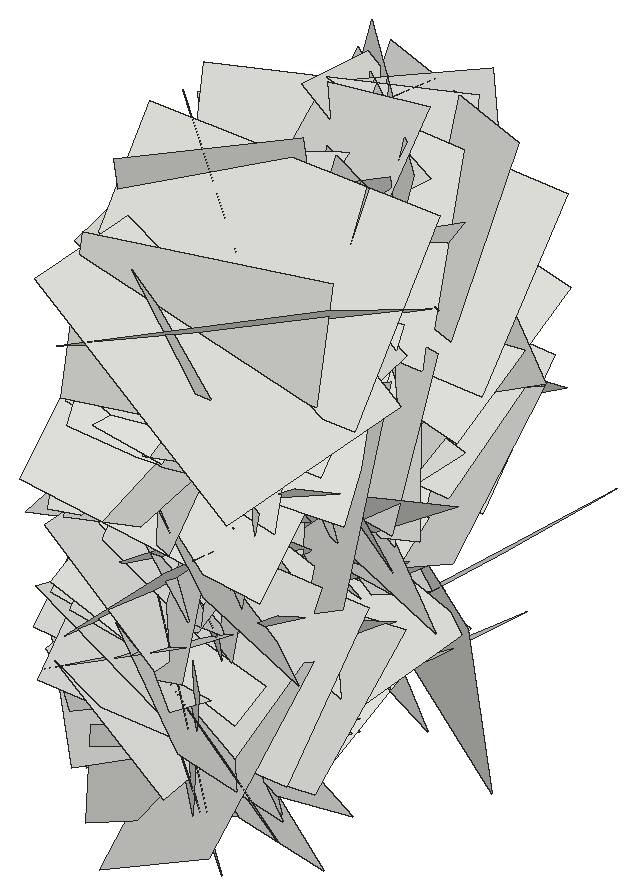
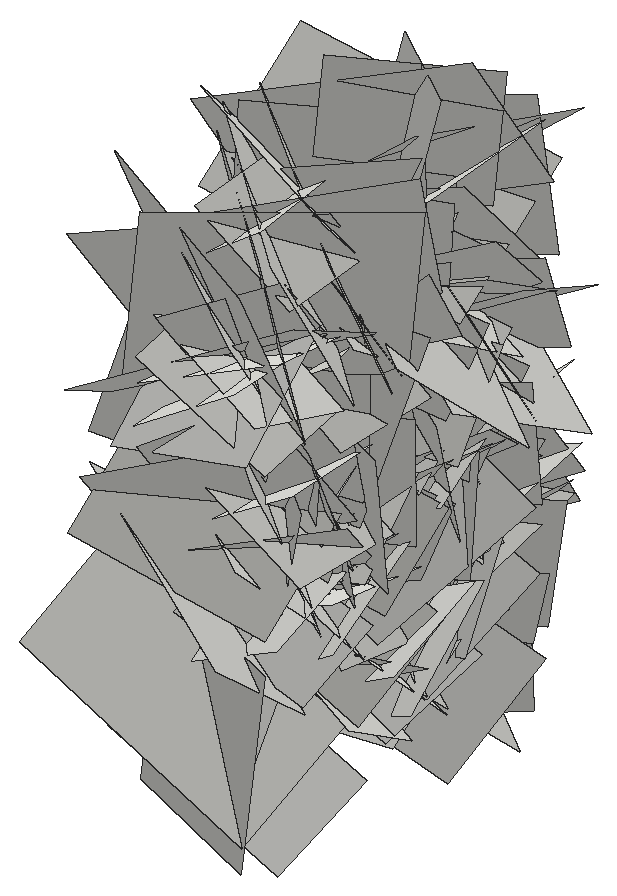
# SketchUp Ruby script. Lengths in inches.
U = 1.inch
M = Sketchup.active_model
def pt(a) = Geom::Point3d.new(a.map { |v| v * U })
def face(e, loops, mat)
  f = e.add_face(loops[0].map { |a| pt(a) })
  loops[1..].each { |l| e.add_face(l.map { |a| pt(a) }).erase! }
  f.material = f.back_material = mat if mat
  f
end
# faces: each face lists its corners as indices into pts; further lists are holes
def faces(e, pts, list, mat = nil) = list.each { |f| face(e, (f[0].is_a?(Array) ? f : [f]).map { |l| l.map { |i| pts[i] } }, mat) }
# xy, xz, yz: faces in a plane at the given z, y or x. An outline is a flat list of corners, or four numbers for a rectangle; further outlines are holes
def ring(l) = l.size == 4 ? [[l[0], l[1]], [l[2], l[1]], [l[2], l[3]], [l[0], l[3]]] : l.each_slice(2).to_a
def flat(e, list, mat, &to3) = list.each { |f| face(e, (f[0].is_a?(Array) ? f : [f]).map { |l| ring(l).map { |u, v| to3.(u, v) } }, mat) }
def xy(e, z, list, mat = nil) = flat(e, list, mat) { |x, y| [x, y, z] }
def xz(e, y, list, mat = nil) = flat(e, list, mat) { |x, z| [x, y, z] }
def yz(e, x, list, mat = nil) = flat(e, list, mat) { |y, z| [x, y, z] }
def lines(e, pts, list) = list.each { |a, b| e.add_line(pt(pts[a]), pt(pts[b])) }
# prism: a flat outline (further loops are holes) pulled along v
def prism(e, loops, v, mat = nil)
  f = face(e, loops, mat); d = Geom::Vector3d.new(v.map { |x| x * U })
  f.pushpull(f.normal.samedirection?(d) ? d.length : -d.length)
end
def box(e, o, s, mat = nil) = prism(e, [[o, [o[0] + s[0], o[1], o[2]], [o[0] + s[0], o[1] + s[1], o[2]], [o[0], o[1] + s[1], o[2]]]], [0, 0, s[2]], mat)
def at(x, y, z, deg = 0) = Geom::Transformation.translation(pt([x, y, z])) * Geom::Transformation.rotation(ORIGIN, Z_AXIS, deg.degrees)
def axes(o, x, y, z) = Geom::Transformation.new([*x, 0, *y, 0, *z, 0, *pt(o).to_a, 1])
def part(name) = M.definitions.add(name)
# library, detail: a bought-in or finely detailed component or shape, given as its bounding box
def library(name, o, s) = part(name).tap { |d| box(d.entities, o, s) }
def detail(e, o, s) = box(e.add_group.entities, o, s)
def put(e, d, t, mat = nil) = e.add_instance(d, t).tap { |i| i.material = mat if mat }
def group(e, t, mat = nil) = e.add_group.tap { |g| g.transformation = t; g.material = mat if mat }.entities
root = M.entities
c1 = part("Component\#6")
p = [[0.01,0,0],[0,3.24,4.54],[4.32,3.24,4.54],[4.33,0,0]]
faces(c1.entities,p,[[0,1,2,3]])
put(root,c1,axes([34.14,168.24,29.62],[-0.00844,-0.1319,-0.59476],[-0.00779,-0.59475,0.132],[0.64572,-0.0089,-0.00618]))
put(root,c1,axes([34.14,163.79,31.02],[-0.0186,-0.39942,0.51021],[-0.04828,0.50989,0.39761],[0.68514,0.02509,0.04187]))
put(root,c1,axes([34.14,167.3,30.05],[-0.09755,-0.36279,0.79394],[-0.2327,0.7823,0.33203],[0.89554,0.16375,0.17276]))
put(root,c1,axes([34.14,166.74,28.03],[-0.20581,0.5378,0.53941],[0.0447,0.5634,-0.54654],[0.80617,0.10606,0.16802]))
put(root,c1,axes([34.14,165.16,26.22],[0.00662,-0.41647,0.48084],[-0.04981,0.47925,0.41571],[0.67246,0.0396,0.02606]))
put(root,c1,axes([38.11,162.15,25.43],[0.09766,0.84172,-0.54191],[-0.18116,-0.52299,-0.84139],[-1.04557,0.16923,0.09516]))
put(root,c1,axes([34.14,170.38,37.22],[-0.01844,-0.65259,0.06973],[-0.0154,0.07012,0.65262],[0.69551,-0.01575,0.0163]))
put(root,c1,axes([38.11,159.15,32.85],[0.28722,0.93511,0.86971],[0.00467,0.88838,-0.95656],[-1.35365,0.20148,0.18123]))
put(root,c1,axes([34.14,158.35,30.49],[-0.08461,0.81055,-0.03501],[-0.12527,-0.04642,-0.80528],[0.85081,0.07377,-0.12204]))
put(root,c1,axes([34.14,168.23,31.98],[-0.11552,-0.73847,0.10601],[0.00435,0.10653,0.74638],[0.79079,-0.10846,0.01138]))
put(root,c1,axes([34.14,162.33,29.83],[-0.22776,0.38392,-0.75072],[0.01782,-0.77261,-0.39993],[0.89361,0.11326,-0.18337]))
put(root,c1,axes([38.11,165.04,27.71],[0.04822,0.07219,0.94774],[-0.14201,0.93984,-0.06516],[-0.99746,-0.13032,0.05509]))
put(root,c1,axes([34.14,171.91,32.4],[0.07209,-0.36069,-0.54144],[-0.07785,-0.54516,0.35394],[0.6852,-0.024,0.09718]))
put(root,c1,axes([38.11,167.29,35.58],[-0.17595,-0.29467,-0.74084],[-0.05215,-0.7515,0.30993],[-0.84352,0.10793,0.13537]))
put(root,c1,axes([38.11,157.3125,32.29],[0.25179,1.05256,0.51222],[-0.06429,0.53303,-1.06718],[-1.23914,0.18623,0.15945]))
put(root,c1,axes([34.14,168.82,35.84],[0.04533,0.37689,0.51175],[-0.01637,0.51337,-0.3768],[0.67349,-0.01289,-0.04361]))
put(root,c1,axes([34.14,159.46,22.85],[-0.09982,-0.0635,0.89488],[-0.1784,0.88507,0.04509],[0.93408,0.16225,0.10424]))
put(root,c1,axes([34.14,160.06,22.6],[-0.02839,-0.24478,0.77995],[-0.15528,0.76918,0.23637],[0.85248,0.13195,0.06903]))
put(root,c1,axes([34.14,159.67,28.14],[-0.12868,0.67272,0.52517],[-0.08613,0.51893,-0.68352],[0.90053,0.14576,0.00967]))
put(root,c1,axes([34.14,158.39,26.84],[-0.02686,0.84806,0.10272],[-0.17857,0.09579,-0.83237],[0.88773,0.04493,-0.16432]))
put(root,c1,axes([34.14,169.17,27.35],[0.00515,-0.4485,-0.48712],[0.04455,-0.48594,0.44784],[0.70046,0.0342,-0.02491]))
put(root,c1,axes([38.11,161.79,25.53],[-0.01152,-0.82607,0.19056],[-0.15176,0.18963,0.81386],[-0.88572,-0.02175,-0.14193]))
put(root,c1,axes([38.11,164.2,31.01],[0.06613,-0.18181,-0.96198],[-0.02897,-0.96387,0.1804],[-1.03734,0.01533,-0.06637]))
put(root,c1,axes([34.14,169.92,30.86],[0.08798,0.07784,-0.70174],[-0.08853,-0.70052,-0.08758],[0.74315,-0.09267,0.07264]))
put(root,c1,axes([38.11,162.32,28.44],[-0.12821,-0.42216,-0.69512],[0.01339,-0.70366,0.42514],[-0.86197,0.05186,0.11]))
put(root,c1,axes([38.11,166.33,22.3],[0.05809,-0.87115,0.26873],[-0.09257,0.26296,0.87026],[-0.96191,-0.07791,-0.06752]))
put(root,c1,axes([38.11,171.77,39.47],[0.25632,-0.1505,-1.28885],[0.2021,-1.29268,0.18672],[-1.36053,-0.22038,-0.21508]))
put(root,c1,axes([34.14,167.69,34.89],[0.01272,-0.59445,-0.3878],[0.01652,-0.38754,0.59453],[0.75216,0.01856,-0.0065]))
put(root,c1,axes([34.14,168.18,25.35],[0.0356,-0.79141,-0.13903],[-0.13499,-0.14264,0.78117],[0.84098,0.01061,0.13127]))
put(root,c1,axes([38.11,163.85,33.45],[0.03445,-0.73428,-0.4148],[-0.17499,-0.41262,0.71747],[-0.87664,0.05351,-0.15952]))
put(root,c1,axes([38.11,158.45,30.92],[0.16236,0.46297,0.88251],[-0.09478,0.89566,-0.45434],[-1.05211,-0.00924,0.17712]))
put(root,c1,axes([38.11,166.53,31.68],[0.02185,0.89564,-0.0065],[-0.05171,-0.00537,-0.89456],[-0.948,0.02094,0.04865]))
put(root,c1,axes([38.11,171.21,38.93],[0.24063,-0.51313,-1.11059],[0.16085,-1.10901,0.54342],[-1.28679,-0.23458,-0.13976]))
put(root,c1,axes([34.14,171.89,34.33],[-0.10287,-0.74562,-0.1631],[0.15609,-0.17961,0.73351],[0.79385,-0.06131,-0.16536]))
put(root,c1,axes([38.11,162.43,26.35],[-0.02315,-0.70596,0.51236],[0.01203,0.51225,0.70629],[-0.92456,0.02434,-0.00364]))
put(root,c1,axes([38.11,162.61,28.57],[0.04222,-0.49534,0.62953],[-0.20196,0.60636,0.48917],[-0.82474,-0.17384,-0.08755]))
put(root,c1,axes([38.11,162.92,24.26],[-0.16568,0.16434,-0.80239],[0.1251,-0.80382,-0.18763],[-0.85913,-0.14874,0.12742]))
put(root,c1,axes([38.11,164.5,23.79],[-0.04443,0.667,0.37408],[-0.11412,0.36576,-0.66423],[-0.80255,-0.08894,0.07374]))
put(root,c1,axes([38.11,168.875,35.8],[-0.07444,0.7996,-0.0855],[-0.00091,-0.0859,-0.80263],[-0.85241,-0.06974,0.00832]))
put(root,c1,axes([34.14,164.96,33.58],[0.03363,-0.67551,-0.53197],[-0.14584,-0.52946,0.66412],[0.89967,-0.06058,0.12754]))
put(root,c1,axes([34.14,169.82,24.93],[0.00586,-0.68753,0.27068],[0.05817,0.27032,0.6855],[0.78107,-0.01497,-0.05308]))
put(root,c1,axes([38.11,164.8,26.41],[-0.06555,-0.88967,-0.10275],[0.1194,-0.1099,0.88381],[-0.94178,0.04799,0.1192]))
put(root,c1,axes([38.11,163.99,40.83],[-0.08038,0.23372,-0.81219],[0.10222,-0.80774,-0.24144],[-0.89001,-0.11388,0.04562]))
put(root,c1,axes([38.11,167.51,23.32],[0.04127,-0.8056,0.43064],[0.05085,0.43224,0.80425],[-0.96695,-0.01165,0.06068]))
put(root,c1,axes([38.11,164.95,29.96],[0.04265,0.57286,-0.52342],[-0.15347,-0.50938,-0.56862],[-0.80809,0.12697,0.08036]))
put(root,c1,axes([34.14,164.95,29.96],[-0.04265,0.57286,-0.52342],[0.15347,-0.50938,-0.56862],[0.80809,0.12697,0.08036]))
put(root,c1,axes([34.14,167.51,23.32],[-0.04127,-0.8056,0.43064],[-0.05085,0.43224,0.80425],[0.96695,-0.01165,0.06068]))
put(root,c1,axes([34.14,163.99,40.83],[0.08038,0.23372,-0.81219],[-0.10222,-0.80774,-0.24144],[0.89001,-0.11388,0.04562]))
put(root,c1,axes([34.14,164.8,26.41],[0.06555,-0.88967,-0.10275],[-0.1194,-0.1099,0.88381],[0.94178,0.04799,0.1192]))
put(root,c1,axes([38.11,169.82,24.93],[-0.00586,-0.68753,0.27068],[-0.05817,0.27032,0.6855],[-0.78107,-0.01497,-0.05308]))
put(root,c1,axes([38.11,164.96,33.58],[-0.03363,-0.67551,-0.53197],[0.14584,-0.52946,0.66412],[-0.89967,-0.06058,0.12754]))
put(root,c1,axes([34.14,168.875,35.8],[0.07444,0.7996,-0.0855],[0.00091,-0.0859,-0.80263],[0.85241,-0.06974,0.00832]))
put(root,c1,axes([34.14,164.5,23.79],[0.04443,0.667,0.37408],[0.11412,0.36576,-0.66423],[0.80255,-0.08894,0.07374]))
put(root,c1,axes([34.14,162.92,24.26],[0.16568,0.16434,-0.80239],[-0.1251,-0.80382,-0.18763],[0.85913,-0.14874,0.12742]))
put(root,c1,axes([34.14,162.61,28.57],[-0.04222,-0.49534,0.62953],[0.20196,0.60636,0.48917],[0.82474,-0.17384,-0.08755]))
put(root,c1,axes([34.14,162.43,26.35],[0.02315,-0.70596,0.51236],[-0.01203,0.51225,0.70629],[0.92456,0.02434,-0.00364]))
put(root,c1,axes([38.11,171.89,34.33],[0.10287,-0.74562,-0.1631],[-0.15609,-0.17961,0.73351],[-0.79385,-0.06131,-0.16536]))
put(root,c1,axes([34.14,171.21,38.93],[-0.24063,-0.51313,-1.11059],[-0.16085,-1.10901,0.54342],[1.28679,-0.23458,-0.13976]))
put(root,c1,axes([34.14,166.53,31.68],[-0.02185,0.89564,-0.0065],[0.05171,-0.00537,-0.89456],[0.948,0.02094,0.04865]))
put(root,c1,axes([34.14,158.45,30.92],[-0.16236,0.46297,0.88251],[0.09478,0.89566,-0.45434],[1.05211,-0.00924,0.17712]))
put(root,c1,axes([34.14,163.85,33.45],[-0.03445,-0.73428,-0.4148],[0.17499,-0.41262,0.71747],[0.87664,0.05351,-0.15952]))
put(root,c1,axes([38.11,168.18,25.35],[-0.0356,-0.79141,-0.13903],[0.13499,-0.14264,0.78117],[-0.84098,0.01061,0.13127]))
put(root,c1,axes([38.11,167.69,34.89],[-0.01272,-0.59445,-0.3878],[-0.01652,-0.38754,0.59453],[-0.75216,0.01856,-0.0065]))
put(root,c1,axes([34.14,171.77,39.47],[-0.25632,-0.1505,-1.28885],[-0.2021,-1.29268,0.18672],[1.36053,-0.22038,-0.21508]))
put(root,c1,axes([34.14,166.33,22.3],[-0.05809,-0.87115,0.26873],[0.09257,0.26296,0.87026],[0.96191,-0.07791,-0.06752]))
put(root,c1,axes([34.14,162.32,28.44],[0.12821,-0.42216,-0.69512],[-0.01339,-0.70366,0.42514],[0.86197,0.05186,0.11]))
put(root,c1,axes([38.11,169.92,30.86],[-0.08798,0.07784,-0.70174],[0.08853,-0.70052,-0.08758],[-0.74315,-0.09267,0.07264]))
put(root,c1,axes([34.14,164.2,31.01],[-0.06613,-0.18181,-0.96198],[0.02897,-0.96387,0.1804],[1.03734,0.01533,-0.06637]))
put(root,c1,axes([34.14,161.79,25.53],[0.01152,-0.82607,0.19056],[0.15176,0.18963,0.81386],[0.88572,-0.02175,-0.14193]))
put(root,c1,axes([38.11,169.17,27.35],[-0.00515,-0.4485,-0.48712],[-0.04455,-0.48594,0.44784],[-0.70046,0.0342,-0.02491]))
put(root,c1,axes([38.11,158.39,26.84],[0.02686,0.84806,0.10272],[0.17857,0.09579,-0.83237],[-0.88773,0.04493,-0.16432]))
put(root,c1,axes([38.11,159.67,28.14],[0.12868,0.67272,0.52517],[0.08613,0.51893,-0.68352],[-0.90053,0.14576,0.00967]))
put(root,c1,axes([38.11,160.06,22.6],[0.02839,-0.24478,0.77995],[0.15528,0.76918,0.23637],[-0.85248,0.13195,0.06903]))
put(root,c1,axes([38.11,159.46,22.85],[0.09982,-0.0635,0.89488],[0.1784,0.88507,0.04509],[-0.93408,0.16225,0.10424]))
put(root,c1,axes([38.11,168.82,35.84],[-0.04533,0.37689,0.51175],[0.01637,0.51337,-0.3768],[-0.67349,-0.01289,-0.04361]))
put(root,c1,axes([34.14,157.3125,32.29],[-0.25179,1.05256,0.51222],[0.06429,0.53303,-1.06718],[1.23914,0.18623,0.15945]))
put(root,c1,axes([34.14,167.29,35.58],[0.17595,-0.29467,-0.74084],[0.05215,-0.7515,0.30993],[0.84352,0.10793,0.13537]))
put(root,c1,axes([38.11,171.91,32.4],[-0.07209,-0.36069,-0.54144],[0.07785,-0.54516,0.35394],[-0.6852,-0.024,0.09718]))
put(root,c1,axes([34.14,165.04,27.71],[-0.04822,0.07219,0.94774],[0.14201,0.93984,-0.06516],[0.99746,-0.13032,0.05509]))
put(root,c1,axes([38.11,162.33,29.83],[0.22776,0.38392,-0.75072],[-0.01782,-0.77261,-0.39993],[-0.89361,0.11326,-0.18337]))
put(root,c1,axes([38.11,168.23,31.98],[0.11552,-0.73847,0.10601],[-0.00435,0.10653,0.74638],[-0.79079,-0.10846,0.01138]))
put(root,c1,axes([38.11,158.35,30.49],[0.08461,0.81055,-0.03501],[0.12527,-0.04642,-0.80528],[-0.85081,0.07377,-0.12204]))
put(root,c1,axes([34.14,159.15,32.85],[-0.28722,0.93511,0.86971],[-0.00467,0.88838,-0.95656],[1.35365,0.20148,0.18123]))
put(root,c1,axes([38.11,170.38,37.22],[0.01844,-0.65259,0.06973],[0.0154,0.07012,0.65262],[-0.69551,-0.01575,0.0163]))
put(root,c1,axes([34.14,162.15,25.43],[-0.09766,0.84172,-0.54191],[0.18116,-0.52299,-0.84139],[1.04557,0.16923,0.09516]))
put(root,c1,axes([38.11,165.16,26.22],[-0.00662,-0.41647,0.48084],[0.04981,0.47925,0.41571],[-0.67246,0.0396,0.02606]))
put(root,c1,axes([38.11,166.74,28.03],[0.20581,0.5378,0.53941],[-0.0447,0.5634,-0.54654],[-0.80617,0.10606,0.16802]))
put(root,c1,axes([38.11,167.3,30.05],[0.09755,-0.36279,0.79394],[0.2327,0.7823,0.33203],[-0.89554,0.16375,0.17276]))
put(root,c1,axes([38.11,163.79,31.02],[0.0186,-0.39942,0.51021],[0.04828,0.50989,0.39761],[-0.68514,0.02509,0.04187]))
put(root,c1,axes([38.11,168.24,29.62],[0.00844,-0.1319,-0.59476],[0.00779,-0.59475,0.132],[-0.64572,-0.0089,-0.00618]))
put(root,c1,axes([34.14,168.37,37.02],[-0.06582,-0.55881,-0.84289],[0.17414,-0.83883,0.54402],[1.05774,0.10333,-0.14201]))
put(root,c1,axes([34.14,162.55,24.47],[0.08094,0.6993,-0.63815],[0.06519,-0.64254,-0.69674],[1.00139,-0.01469,0.09694]))
put(root,c1,axes([38.11,167.47,38.84],[0.19203,-0.25676,-0.78485],[0.09527,-0.79261,0.28005],[-0.87013,-0.14344,-0.14255]))
put(root,c1,axes([38.11,168.14,25.37],[0.00005,-0.54267,0.44601],[0.16088,0.43548,0.52984],[-0.72699,0.09633,0.11728]))
put(root,c1,axes([34.14,169.13,31.47],[0.22896,-0.22184,-0.76377],[0.12794,-0.77313,0.25869],[0.83329,0.17965,0.17014]))
put(root,c1,axes([34.14,164.67,22.86],[-0.07455,-1.03669,0.46758],[0.01691,0.46753,1.03897],[1.20537,-0.07068,0.01434]))
put(root,c1,axes([38.11,161.42,33.85],[0.12931,-0.58697,0.4315],[0.06321,0.44408,0.58723],[-0.76963,-0.06214,0.12073]))
put(root,c1,axes([34.14,160.7,27.63],[-0.09928,0.64406,-0.88513],[0.13228,-0.87629,-0.65083],[1.15276,0.15602,-0.00154]))
put(root,c1,axes([34.14,159.57,38.3125],[-0.19748,1.37219,0.09956],[-0.15298,0.08042,-1.37849],[1.4503,0.19533,-0.13185]))
put(root,c1,axes([38.11,165.91,24.52],[-0.03596,-0.58924,0.24858],[0.15481,0.23521,0.57749],[-0.65999,0.08727,0.12191]))
put(root,c1,axes([34.14,166.55,31.56],[0.0814,0.41102,-0.8284],[0.17089,-0.82447,-0.39413],[0.96524,0.11131,0.13964]))
put(root,c1,axes([38.11,169.1,21.1],[0.05323,-0.42134,0.48328],[0.06346,0.48572,0.41725],[-0.67666,0.01241,0.07715]))
put(root,c1,axes([34.14,166.67,25.47],[-0.29316,-1.18227,0.54308],[0.10516,0.53443,1.21398],[1.37509,-0.29293,0.02294]))
put(root,c1,axes([34.14,168.75,37.98],[-0.06882,-0.53698,-1.12739],[-0.1022,-1.12338,0.54063],[1.31971,-0.115,-0.01692]))
put(root,c1,axes([34.14,158.58,28.72],[0.17742,0.80309,0.64454],[-0.10421,0.66248,-0.79991],[1.08655,-0.0676,-0.18196]))
put(root,c1,axes([38.11,163.1,21.29],[0.03251,-0.459,0.52355],[0.17075,0.51451,0.44164],[-0.71801,0.10157,0.12873]))
put(root,c1,axes([34.14,169.04,36.23],[-0.04162,0.78981,-0.64322],[0.24351,-0.62024,-0.77563],[1.05189,0.17484,0.15411]))
put(root,c1,axes([34.14,170.89,20.28],[0.12274,-1.02279,0.17958],[-0.0333,0.17716,1.02926],[1.10024,0.11946,0.01112]))
put(root,c1,axes([34.14,167.53,29.6],[0.04916,0.6172,0.8297],[0.08211,0.82613,-0.61887],[1.09305,-0.08981,0.00917]))
put(root,c1,axes([34.14,171.44,27.64],[0.05126,-0.8571,0.56567],[0.11133,0.56746,0.85083],[1.08285,-0.01777,-0.11425]))
put(root,c1,axes([38.11,163.13,28.77],[0.13219,-0.55975,0.33448],[0.05965,0.34851,0.56225],[-0.68862,-0.07726,0.11291]))
put(root,c1,axes([34.14,163.625,35.04],[0.27654,-0.44632,0.88094],[-0.09901,0.89592,0.48157],[1.04211,0.20356,-0.18801]))
put(root,c1,axes([34.14,167.41,29.34],[-0.20833,-0.42173,1.22713],[0.0869,1.23461,0.43743],[1.37269,-0.14217,0.15855]))
put(root,c1,axes([34.14,168.84,39.14],[0.0295,-0.69575,-0.73723],[0.22295,-0.71749,0.68506],[1.05113,0.17171,-0.12461]))
put(root,c1,axes([34.14,163.85,26.9],[0.03329,1.04875,0.11229],[0.24045,0.10299,-1.02538],[1.09187,-0.05466,0.22238]))
put(root,c1,axes([34.14,160.22,28.4],[0.15479,0.80897,-0.76348],[-0.02106,-0.76802,-0.81757],[1.17891,-0.11994,0.08565]))
put(root,c1,axes([34.14,169.63,32.59],[0.01533,-0.4611,-1.03377],[0.17767,-1.02158,0.45801],[1.18663,0.15892,-0.05522]))
put(root,c1,axes([34.14,159.8,34.2],[-0.03301,0.77795,0.85676],[0.24326,0.8442,-0.75821],[1.20233,-0.14944,0.17692]))
put(root,c1,axes([34.14,166.97,25.06],[-0.03339,-0.82276,-0.77538],[0.30966,-0.75526,0.78954],[1.15769,0.17829,-0.23355]))
put(root,c1,axes([34.14,165.55,34.43],[-0.04885,1.13911,0.54464],[0.08516,0.54654,-1.13629],[1.33566,0.00681,0.09237]))
put(root,c1,axes([34.14,164.92,23.28],[0.02573,-1.02703,-0.88101],[-0.12942,-0.87922,1.02158],[1.42847,-0.06116,0.10843]))
put(root,c1,axes([34.14,160.96,32.62],[0.12215,0.75895,-0.88724],[0.014,-0.89234,-0.7616],[1.23753,-0.06482,0.09619]))
put(root,c1,axes([34.14,172.54,38.57],[-0.12011,-0.4932,-1.18141],[0.20578,-1.17893,0.47355],[1.34134,0.1367,-0.17844]))
put(root,c1,axes([34.14,171.44,26.6],[-0.03428,0.27698,-1.26013],[0.06702,-1.25867,-0.27828],[1.36598,0.0687,-0.01797]))
put(root,c1,axes([34.14,173.53,27.66],[0.08068,-0.97468,-0.75893],[0.01331,-0.75972,0.97695],[1.30935,0.06778,0.03684]))
put(root,c1,axes([34.14,158.99,33.95],[0.09747,0.08794,1.12692],[0.17247,1.11783,-0.1005],[1.18568,-0.16983,-0.07802]))
put(root,c1,axes([34.14,166.62,31.96],[0.21061,0.75098,-0.921],[-0.02022,-0.93165,-0.76377],[1.25951,-0.14053,0.14175]))
put(root,c1,axes([34.14,158.06,26.05],[0.19995,0.52409,1.06255],[0.00833,1.07535,-0.5318],[1.25583,-0.09057,-0.16565]))
put(root,c1,axes([34.14,172.42,21.79],[0.22827,-1.35966,0.24048],[-0.1567,0.21929,1.3722],[1.45519,0.2369,0.11004]))
put(root,c1,axes([34.14,165.11,34.6875],[0.03998,0.77126,1.05992],[0.2457,1.03973,-0.76482],[1.36759,-0.20934,0.10642]))
put(root,c1,axes([34.14,159.18,36.25],[0.04304,0.74935,1.15311],[0.14712,1.14549,-0.74928],[1.45028,-0.13844,0.04179]))
put(root,c1,axes([34.14,168.45,29.92],[0.2904,-0.81126,-1.09363],[-0.15157,-1.12651,0.79984],[1.4354,0.04517,0.30571]))
put(root,c1,axes([34.14,157.9,37.93],[0.24747,1.3445,0.30187],[-0.11522,0.32319,-1.35538],[1.4561,-0.20293,-0.15855]))
put(root,c1,axes([34.14,163.2,33.68],[0.16473,-1.2102,0.57798],[0.2383,0.59712,1.18983],[1.40149,0.04071,-0.27024]))
